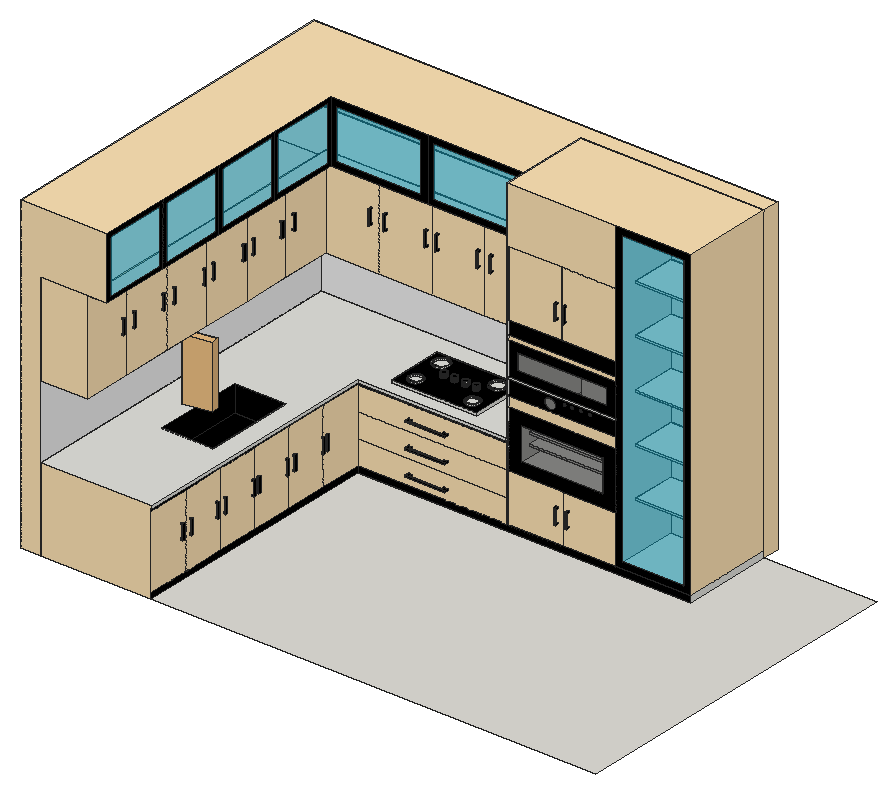
# SketchUp Ruby script. Lengths in inches.
U = 1.inch
M = Sketchup.active_model
def pt(a) = Geom::Point3d.new(a.map { |v| v * U })
def face(e, loops, mat)
  f = e.add_face(loops[0].map { |a| pt(a) })
  loops[1..].each { |l| e.add_face(l.map { |a| pt(a) }).erase! }
  f.material = f.back_material = mat if mat
  f
end
# faces: each face lists its corners as indices into pts; further lists are holes
def faces(e, pts, list, mat = nil) = list.each { |f| face(e, (f[0].is_a?(Array) ? f : [f]).map { |l| l.map { |i| pts[i] } }, mat) }
# xy, xz, yz: faces in a plane at the given z, y or x. An outline is a flat list of corners, or four numbers for a rectangle; further outlines are holes
def ring(l) = l.size == 4 ? [[l[0], l[1]], [l[2], l[1]], [l[2], l[3]], [l[0], l[3]]] : l.each_slice(2).to_a
def flat(e, list, mat, &to3) = list.each { |f| face(e, (f[0].is_a?(Array) ? f : [f]).map { |l| ring(l).map { |u, v| to3.(u, v) } }, mat) }
def xy(e, z, list, mat = nil) = flat(e, list, mat) { |x, y| [x, y, z] }
def xz(e, y, list, mat = nil) = flat(e, list, mat) { |x, z| [x, y, z] }
def yz(e, x, list, mat = nil) = flat(e, list, mat) { |y, z| [x, y, z] }
def lines(e, pts, list) = list.each { |a, b| e.add_line(pt(pts[a]), pt(pts[b])) }
# prism: a flat outline (further loops are holes) pulled along v
def prism(e, loops, v, mat = nil)
  f = face(e, loops, mat); d = Geom::Vector3d.new(v.map { |x| x * U })
  f.pushpull(f.normal.samedirection?(d) ? d.length : -d.length)
end
def box(e, o, s, mat = nil) = prism(e, [[o, [o[0] + s[0], o[1], o[2]], [o[0] + s[0], o[1] + s[1], o[2]], [o[0], o[1] + s[1], o[2]]]], [0, 0, s[2]], mat)
def at(x, y, z, deg = 0) = Geom::Transformation.translation(pt([x, y, z])) * Geom::Transformation.rotation(ORIGIN, Z_AXIS, deg.degrees)
def axes(o, x, y, z) = Geom::Transformation.new([*x, 0, *y, 0, *z, 0, *pt(o).to_a, 1])
def part(name) = M.definitions.add(name)
# library, detail: a bought-in or finely detailed component or shape, given as its bounding box
def library(name, o, s) = part(name).tap { |d| box(d.entities, o, s) }
def detail(e, o, s) = box(e.add_group.entities, o, s)
def put(e, d, t, mat = nil) = e.add_instance(d, t).tap { |i| i.material = mat if mat }
def group(e, t, mat = nil) = e.add_group.tap { |g| g.transformation = t; g.material = mat if mat }.entities
root = M.entities
M.materials.add("[0032_Moccasin]").color = [255, 228, 181]
M.materials.add("[0137_Black]").color = [0, 0, 0]
M.materials.add("[Carrera Marble]").color = [239, 239, 239]
M.materials.add("[Marble Carrara Gold Floor Tile]").color = [225, 223, 217]
M.materials.add("[Translucent Glass Gray]").color = [53, 53, 53]
M.materials["[Translucent Glass Gray]"].alpha = 0.5
M.materials.add("[Translucent Glass Tinted]").color = [7, 187, 224]
M.materials["[Translucent Glass Tinted]"].alpha = 0.48
c1 = part("Group\#2")
xy(c1.entities,0,[[0,0,0.375,0.22]])
xy(c1.entities,0.1875,[[0,0,0.27,0.22]])
xy(c1.entities,1.75,[[0,0,0.27,0.22]])
xy(c1.entities,1.9375,[[0,0,0.375,0.22]])
xz(c1.entities,0,[[0,0,0.375,0,0.375,1.9375,0,1.9375,0,1.75,0.27,1.75,0.27,0.1875,0,0.1875]])
xz(c1.entities,0.22,[[0,0,0,0.1875,0.27,0.1875,0.27,1.75,0,1.75,0,1.9375,0.375,1.9375,0.375,0]])
yz(c1.entities,0.27,[[0,0.1875,0.22,1.75]])
yz(c1.entities,0.375,[[0,0,0.22,1.9375]])
c2 = library("Group\#3",[0,0,0],[12,29.06,81.36])
xy(root,0,[[0,0,0,46.44,58.57,46.44,58.57,44.34,2.55,44.34,2.55,0],[2.55,0,2.55,44.34,58.57,44.34,58.57,32.6875,16.51,32.6875,16.51,0]])
xy(root,0,[[16.51,0,72.74,0,72.74,44.34,58.57,44.34,58.57,32.6875,16.51,32.6875]],"[Marble Carrara Gold Floor Tile]")
xy(root,0.74,[[35.38,32.6875,58.57,44.34]])
xy(root,1.6,[[50.01,32.6875,57.71,40.25]])
xy(root,7.25,[[7.58,12.86,14.08,24.36]],"[0137_Black]")
xy(root,7.76,[[50.01,34.625,57.71,40.25]])
xy(root,7.99,[[50.01,34.625,57.71,40.25]])
xy(root,8.47,[[37.24,32.6875,47.54,36.6875]])
xy(root,9.82,[[37.24,33.8125,47.54,36.6875]])
xy(root,10.05,[[37.24,33.8125,47.54,36.6875]])
xy(root,10.25,[[16.51,0,16.51,32.6875,35.38,32.6875,35.38,32.5625,16.64,32.5625,16.64,0]])
xy(root,10.5625,[[[2.55,0,16.64,0,16.64,32.5625,35.38,32.5625,35.38,44.34,2.55,44.34],[19.61,34.25,30.3,41.32],[7.58,12.86,14.08,24.36]],[19.61,34.25,30.3,41.32]])
xy(root,10.9375,[[[21.41,34.87,21.19,34.9,20.97,34.99,20.79,35.125,20.65,35.31,20.57,35.52,20.54,35.74,20.57,35.97,20.65,36.18,20.79,36.36,20.97,36.5,21.19,36.59,21.41,36.62,21.64,36.59,21.85,36.5,22.03,36.36,22.17,36.18,22.26,35.97,22.29,35.74,22.26,35.52,22.17,35.31,22.03,35.125,21.85,34.99,21.64,34.9],[21.41,35.04,21.59,35.07,21.76,35.14,21.91,35.25,22.02,35.39,22.09,35.5625,22.11,35.74,22.09,35.92,22.02,36.09,21.91,36.24,21.76,36.35,21.59,36.42,21.41,36.44,21.23,36.42,21.0625,36.35,20.92,36.24,20.8,36.09,20.73,35.92,20.71,35.74,20.73,35.5625,20.8,35.39,20.92,35.25,21.0625,35.14,21.23,35.07]],[[28.6,34.87,28.375,34.9,28.16,34.99,27.98,35.125,27.84,35.31,27.75,35.52,27.72,35.74,27.75,35.97,27.84,36.18,27.98,36.36,28.16,36.5,28.375,36.59,28.6,36.62,28.83,36.59,29.04,36.5,29.22,36.36,29.36,36.18,29.44,35.97,29.47,35.74,29.44,35.52,29.36,35.31,29.22,35.125,29.04,34.99,28.83,34.9],[28.6,35.0625,28.78,35.08,28.94,35.15,29.08,35.26,29.19,35.4,29.26,35.57,29.28,35.74,29.26,35.92,29.19,36.08,29.08,36.22,28.94,36.33,28.78,36.4,28.6,36.42,28.42,36.4,28.26,36.33,28.12,36.22,28.01,36.08,27.94,35.92,27.92,35.74,27.94,35.57,28.01,35.4,28.12,35.26,28.26,35.15,28.42,35.08]],[21.41,35.04,21.59,35.07,21.76,35.14,21.91,35.25,22.02,35.39,22.09,35.5625,22.11,35.74,22.09,35.92,22.02,36.09,21.91,36.24,21.76,36.35,21.59,36.42,21.41,36.44,21.23,36.42,21.0625,36.35,20.92,36.24,20.8,36.09,20.73,35.92,20.71,35.74,20.73,35.5625,20.8,35.39,20.92,35.25,21.0625,35.14,21.23,35.07],[28.6,35.0625,28.78,35.08,28.94,35.15,29.08,35.26,29.19,35.4,29.26,35.57,29.28,35.74,29.26,35.92,29.19,36.08,29.08,36.22,28.94,36.33,28.78,36.4,28.6,36.42,28.42,36.4,28.26,36.33,28.12,36.22,28.01,36.08,27.94,35.92,27.92,35.74,27.94,35.57,28.01,35.4,28.12,35.26,28.26,35.15,28.42,35.08],[23.23,37.54,23.14,37.56,23.05,37.59,22.97,37.65,22.91,37.73,22.87,37.82,22.86,37.92,22.87,38.02,22.91,38.11,22.97,38.18,23.05,38.24,23.14,38.28,23.23,38.29,23.33,38.28,23.42,38.24,23.5,38.18,23.56,38.11,23.6,38.02,23.61,37.92,23.6,37.82,23.56,37.73,23.5,37.65,23.42,37.59,23.33,37.56],
  [24.56,37.54,24.46,37.56,24.37,37.59,24.29,37.65,24.23,37.73,24.2,37.82,24.18,37.92,24.2,38.02,24.23,38.11,24.29,38.18,24.37,38.24,24.46,38.28,24.56,38.29,24.65,38.28,24.74,38.24,24.82,38.18,24.88,38.11,24.92,38.02,24.93,37.92,24.92,37.82,24.88,37.73,24.82,37.65,24.74,37.59,24.65,37.56],[25.95,37.54,25.85,37.56,25.76,37.6,25.6875,37.66,25.63,37.74,25.59,37.83,25.58,37.93,25.6,38.03,25.64,38.12,25.7,38.19,25.78,38.25,25.87,38.28,25.97,38.29,26.07,38.28,26.16,38.24,26.23,38.18,26.29,38.1,26.32,38.01,26.33,37.91,26.32,37.8125,26.28,37.72,26.22,37.65,26.14,37.59,26.05,37.55],[27.3125,37.55,27.22,37.57,27.13,37.6,27.06,37.66,27,37.74,26.96,37.82,26.95,37.92,26.96,38.01,27,38.1,27.06,38.18,27.13,38.23,27.22,38.27,27.3125,38.28,27.41,38.27,27.5,38.23,27.57,38.18,27.63,38.1,27.67,38.01,27.68,37.92,27.67,37.82,27.63,37.74,27.57,37.66,27.5,37.6,27.41,37.57],[[28.67,38.77,28.41,38.79,28.17,38.87,27.95,39.01,27.77,39.21,27.66,39.44,27.6,39.7,27.62,39.96,27.7,40.21,27.84,40.42,28.04,40.6,28.27,40.72,28.53,40.77,28.79,40.75,29.03,40.67,29.25,40.53,29.43,40.33,29.54,40.1,29.6,39.85,29.58,39.59,29.5,39.34,29.36,39.12,29.16,38.95,28.93,38.83],[28.66,38.97,28.87,39.01,29.05,39.11,29.21,39.25,29.33,39.42,29.39,39.62,29.4,39.83,29.36,40.04,29.27,40.23,29.125,40.38,28.95,40.5,28.75,40.5625,28.54,40.58,28.33,40.53,28.15,40.4375,27.99,40.3,27.875,40.12,27.81,39.92,27.8,39.71,27.84,39.51,27.93,39.32,28.07,39.16,28.25,39.05,28.45,38.98]],[[21.27,38.78,21.02,38.85,20.79,38.99,20.61,39.17,20.48,39.4,20.42,39.65,20.42,39.91,20.49,40.16,20.625,40.39,20.8125,40.57,21.04,40.7,21.29,40.76,21.55,40.76,21.8,40.69,22.03,40.56,22.21,40.37,22.34,40.14,22.4,39.89,22.4,39.63,22.33,39.38,22.2,39.15,22.01,38.97,21.78,38.84,21.53,38.78],[21.29,38.95,21.51,38.95,21.72,39,21.91,39.11,22.0625,39.26,22.17,39.45,22.23,39.66,22.23,39.87,22.18,40.08,22.07,40.27,21.92,40.42,21.74,40.53,21.53,40.59,21.3125,40.59,21.1,40.54,20.92,40.43,20.76,40.28,20.65,40.1,20.59,39.89,20.59,39.67,20.64,39.46,20.75,39.28,20.9,39.12,21.09,39.01]],
  [21.29,38.95,21.51,38.95,21.72,39,21.91,39.11,22.0625,39.26,22.17,39.45,22.23,39.66,22.23,39.87,22.18,40.08,22.07,40.27,21.92,40.42,21.74,40.53,21.53,40.59,21.3125,40.59,21.1,40.54,20.92,40.43,20.76,40.28,20.65,40.1,20.59,39.89,20.59,39.67,20.64,39.46,20.75,39.28,20.9,39.12,21.09,39.01],[28.66,38.97,28.87,39.01,29.05,39.11,29.21,39.25,29.33,39.42,29.39,39.62,29.4,39.83,29.36,40.04,29.27,40.23,29.125,40.38,28.95,40.5,28.75,40.5625,28.54,40.58,28.33,40.53,28.15,40.4375,27.99,40.3,27.875,40.12,27.81,39.92,27.8,39.71,27.84,39.51,27.93,39.32,28.07,39.16,28.25,39.05,28.45,38.98]])
xy(root,10.9375,[[[19.61,34.25,30.3,41.32],[28.67,38.77,28.41,38.79,28.17,38.87,27.95,39.01,27.77,39.21,27.66,39.44,27.6,39.7,27.62,39.96,27.7,40.21,27.84,40.42,28.04,40.6,28.27,40.72,28.53,40.77,28.79,40.75,29.03,40.67,29.25,40.53,29.43,40.33,29.54,40.1,29.6,39.85,29.58,39.59,29.5,39.34,29.36,39.12,29.16,38.95,28.93,38.83],[21.27,38.78,21.02,38.85,20.79,38.99,20.61,39.17,20.48,39.4,20.42,39.65,20.42,39.91,20.49,40.16,20.625,40.39,20.8125,40.57,21.04,40.7,21.29,40.76,21.55,40.76,21.8,40.69,22.03,40.56,22.21,40.37,22.34,40.14,22.4,39.89,22.4,39.63,22.33,39.38,22.2,39.15,22.01,38.97,21.78,38.84,21.53,38.78],[21.41,34.87,21.19,34.9,20.97,34.99,20.79,35.125,20.65,35.31,20.57,35.52,20.54,35.74,20.57,35.97,20.65,36.18,20.79,36.36,20.97,36.5,21.19,36.59,21.41,36.62,21.64,36.59,21.85,36.5,22.03,36.36,22.17,36.18,22.26,35.97,22.29,35.74,22.26,35.52,22.17,35.31,22.03,35.125,21.85,34.99,21.64,34.9],[28.6,34.87,28.375,34.9,28.16,34.99,27.98,35.125,27.84,35.31,27.75,35.52,27.72,35.74,27.75,35.97,27.84,36.18,27.98,36.36,28.16,36.5,28.375,36.59,28.6,36.62,28.83,36.59,29.04,36.5,29.22,36.36,29.36,36.18,29.44,35.97,29.47,35.74,29.44,35.52,29.36,35.31,29.22,35.125,29.04,34.99,28.83,34.9],[25.95,37.54,25.85,37.56,25.76,37.6,25.6875,37.66,25.63,37.74,25.59,37.83,25.58,37.93,25.6,38.03,25.64,38.12,25.7,38.19,25.78,38.25,25.87,38.28,25.97,38.29,26.07,38.28,26.16,38.24,26.23,38.18,26.29,38.1,26.32,38.01,26.33,37.91,26.32,37.8125,26.28,37.72,26.22,37.65,26.14,37.59,26.05,37.55],[23.23,37.54,23.14,37.56,23.05,37.59,22.97,37.65,22.91,37.73,22.87,37.82,22.86,37.92,22.87,38.02,22.91,38.11,22.97,38.18,23.05,38.24,23.14,38.28,23.23,38.29,23.33,38.28,23.42,38.24,23.5,38.18,23.56,38.11,23.6,38.02,23.61,37.92,23.6,37.82,23.56,37.73,23.5,37.65,23.42,37.59,23.33,37.56],[24.56,37.54,24.46,37.56,24.37,37.59,24.29,37.65,24.23,37.73,24.2,37.82,24.18,37.92,24.2,38.02,24.23,38.11,24.29,38.18,24.37,38.24,24.46,38.28,24.56,38.29,24.65,38.28,24.74,38.24,24.82,38.18,24.88,38.11,24.92,38.02,24.93,37.92,24.92,37.82,24.88,37.73,24.82,37.65,24.74,37.59,24.65,37.56],[27.3125,37.55,27.22,37.57,27.13,37.6,27.06,37.66,27,37.74,26.96,37.82,26.95,37.92,26.96,38.01,27,38.1,27.06,38.18,27.13,38.23,27.22,38.27,27.3125,38.28,27.41,38.27,27.5,38.23,27.57,38.18,27.63,38.1,27.67,38.01,27.68,37.92,27.67,37.82,27.63,37.74,27.57,37.66,27.5,37.6,27.41,37.57]]],"[0137_Black]")
xy(root,11.0625,[[[21.41,34.87,21.64,34.9,21.85,34.99,22.03,35.125,22.17,35.31,22.26,35.52,22.29,35.74,22.26,35.97,22.17,36.18,22.03,36.36,21.85,36.5,21.64,36.59,21.41,36.62,21.19,36.59,20.97,36.5,20.79,36.36,20.65,36.18,20.57,35.97,20.54,35.74,20.57,35.52,20.65,35.31,20.79,35.125,20.97,34.99,21.19,34.9],[21.41,35.04,21.23,35.07,21.0625,35.14,20.92,35.25,20.8,35.39,20.73,35.5625,20.71,35.74,20.73,35.92,20.8,36.09,20.92,36.24,21.0625,36.35,21.23,36.42,21.41,36.44,21.59,36.42,21.76,36.35,21.91,36.24,22.02,36.09,22.09,35.92,22.11,35.74,22.09,35.5625,22.02,35.39,21.91,35.25,21.76,35.14,21.59,35.07]],[[28.6,34.87,28.83,34.9,29.04,34.99,29.22,35.125,29.36,35.31,29.44,35.52,29.47,35.74,29.44,35.97,29.36,36.18,29.22,36.36,29.04,36.5,28.83,36.59,28.6,36.62,28.375,36.59,28.16,36.5,27.98,36.36,27.84,36.18,27.75,35.97,27.72,35.74,27.75,35.52,27.84,35.31,27.98,35.125,28.16,34.99,28.375,34.9],[28.6,35.0625,28.42,35.08,28.26,35.15,28.12,35.26,28.01,35.4,27.94,35.57,27.92,35.74,27.94,35.92,28.01,36.08,28.12,36.22,28.26,36.33,28.42,36.4,28.6,36.42,28.78,36.4,28.94,36.33,29.08,36.22,29.19,36.08,29.26,35.92,29.28,35.74,29.26,35.57,29.19,35.4,29.08,35.26,28.94,35.15,28.78,35.08]],[[28.67,38.77,28.93,38.83,29.16,38.95,29.36,39.12,29.5,39.34,29.58,39.59,29.6,39.85,29.54,40.1,29.43,40.33,29.25,40.53,29.03,40.67,28.79,40.75,28.53,40.77,28.27,40.72,28.04,40.6,27.84,40.42,27.7,40.21,27.62,39.96,27.6,39.7,27.66,39.44,27.77,39.21,27.95,39.01,28.17,38.87,28.41,38.79],[28.66,38.97,28.45,38.98,28.25,39.05,28.07,39.16,27.93,39.32,27.84,39.51,27.8,39.71,27.81,39.92,27.875,40.12,27.99,40.3,28.15,40.4375,28.33,40.53,28.54,40.58,28.75,40.5625,28.95,40.5,29.125,40.38,29.27,40.23,29.36,40.04,29.4,39.83,29.39,39.62,29.33,39.42,29.21,39.25,29.05,39.11,28.87,39.01]],[[21.27,38.78,21.53,38.78,21.78,38.84,22.01,38.97,22.2,39.15,22.33,39.38,22.4,39.63,22.4,39.89,22.34,40.14,22.21,40.37,22.03,40.56,21.8,40.69,21.55,40.76,21.29,40.76,21.04,40.7,20.8125,40.57,20.625,40.39,20.49,40.16,20.42,39.91,20.42,39.65,20.48,39.4,20.61,39.17,20.79,38.99,21.02,38.85],[21.29,38.95,21.09,39.01,20.9,39.12,20.75,39.28,20.64,39.46,20.59,39.67,20.59,39.89,20.65,40.1,20.76,40.28,20.92,40.43,21.1,40.54,21.3125,40.59,21.53,40.59,21.74,40.53,21.92,40.42,22.07,40.27,22.18,40.08,22.23,39.87,22.23,39.66,22.17,39.45,22.0625,39.26,21.91,39.11,21.72,39,21.51,38.95]]],"[0137_Black]")
xy(root,11.16,[[37.24,33.8125,47.54,36.6875]])
xy(root,11.36,[[37.24,33.8125,47.54,36.6875]])
xy(root,11.4375,[[23.23,37.54,23.33,37.56,23.42,37.59,23.5,37.65,23.56,37.73,23.6,37.82,23.61,37.92,23.6,38.02,23.56,38.11,23.5,38.18,23.42,38.24,23.33,38.28,23.23,38.29,23.14,38.28,23.05,38.24,22.97,38.18,22.91,38.11,22.87,38.02,22.86,37.92,22.87,37.82,22.91,37.73,22.97,37.65,23.05,37.59,23.14,37.56],[24.56,37.54,24.65,37.56,24.74,37.59,24.82,37.65,24.88,37.73,24.92,37.82,24.93,37.92,24.92,38.02,24.88,38.11,24.82,38.18,24.74,38.24,24.65,38.28,24.56,38.29,24.46,38.28,24.37,38.24,24.29,38.18,24.23,38.11,24.2,38.02,24.18,37.92,24.2,37.82,24.23,37.73,24.29,37.65,24.37,37.59,24.46,37.56],[25.95,37.54,26.05,37.55,26.14,37.59,26.22,37.65,26.28,37.72,26.32,37.8125,26.33,37.91,26.32,38.01,26.29,38.1,26.23,38.18,26.16,38.24,26.07,38.28,25.97,38.29,25.87,38.28,25.78,38.25,25.7,38.19,25.64,38.12,25.6,38.03,25.58,37.93,25.59,37.83,25.63,37.74,25.6875,37.66,25.76,37.6,25.85,37.56],[27.3125,37.55,27.41,37.57,27.5,37.6,27.57,37.66,27.63,37.74,27.67,37.82,27.68,37.92,27.67,38.01,27.63,38.1,27.57,38.18,27.5,38.23,27.41,38.27,27.3125,38.28,27.22,38.27,27.13,38.23,27.06,38.18,27,38.1,26.96,38.01,26.95,37.92,26.96,37.82,27,37.74,27.06,37.66,27.13,37.6,27.22,37.57]],"[0137_Black]")
xy(root,12.51,[[37.24,32.6875,47.54,36.6875]])
xy(root,13.91,[[50.01,34.625,57.71,40.25]])
xy(root,14.15,[[50.01,34.625,57.71,40.25]])
xy(root,19.85,[[2.55,0,2.55,44.34,35.38,44.34,35.38,37.65,8.49,37.65,8.49,0]])
xy(root,20.06,[[50.01,34.625,57.71,40.25]])
xy(root,20.3,[[50.01,34.625,57.71,40.25]])
xy(root,24.01,[[35.56,32.6875,35.64,32.75],[42.25,32.6875,42.28,32.75]])
xy(root,26.21,[[50.01,34.625,57.71,40.25]])
xy(root,26.45,[[50.01,34.625,57.71,40.25]])
xy(root,31.56,[[2.55,0,8.49,36.47],[8.49,0,8.49,37.65,35.38,37.65,35.38,35.34,10.99,35.34,10.99,0],[2.55,36.47,8.49,36.47,8.49,37.65,35.38,37.65,35.38,44.34,2.55,44.34]])
xy(root,32.29,[[35.56,32.6875,35.64,32.75],[42.25,32.6875,42.28,32.75]])
xy(root,32.36,[[50.01,34.625,57.71,40.25]])
xy(root,32.6,[[50.01,34.625,57.71,40.25]])
xy(root,38.51,[[50.01,32.6875,57.71,40.25]])
xy(root,39.375,[[0,0,10.99,0,10.99,35.34,35.38,35.34,35.38,44.34,58.57,44.34,58.57,46.44,0,46.44],[35.38,32.6875,58.57,44.34]],"[0032_Moccasin]")
xz(root,0,[[0,0,2.55,0,2.55,31.56,10.99,31.56,10.99,39.375,0,39.375],[2.55,0,16.51,0,16.51,10.25,16.64,10.25,16.64,10.5625,2.55,10.5625],[2.55,19.85,8.49,31.56]],"[0032_Moccasin]")
xz(root,12.86,[[7.58,7.25,14.08,10.5625]],"[0137_Black]")
xz(root,24.36,[[7.58,7.25,14.08,10.5625]],"[0137_Black]")
xz(root,32.5625,[[16.64,10.25,35.38,10.5625]])
xz(root,32.6875,[[35.38,0.74,35.64,24.01],[35.64,17.33,49.14,17.52],[35.38,24.01,35.56,32.29]])
xz(root,32.6875,[[16.51,0.74,35.38,3.8],[35.64,0.74,42.39,6.86],[42.39,0.74,49.14,6.86],[16.51,3.8,35.38,6.86],[16.51,6.86,35.38,9.92],
  [35.64,14.11,49.14,15.4375],[35.64,21.77,49.14,22.3],[35.64,24.01,42.25,32.29],[42.28,24.01,49.14,32.29],[35.38,32.29,49.14,39.375]],"[0032_Moccasin]")
xz(root,32.6875,[[16.51,0,58.57,0.74],[[49.14,0.74,58.57,39.375],[50.01,1.6,57.71,38.51]],[[35.64,6.86,49.14,14.11],[37.24,8.47,47.54,12.51]],[16.51,9.92,35.38,10.25],[[35.64,15.4375,49.14,17.33],[40.85,15.62,40.68,15.64,40.51,15.71,40.37,15.82,40.26,15.96,40.1875,16.13,40.17,16.31,40.1875,16.49,40.26,16.65,40.37,16.79,40.51,16.9,40.68,16.97,40.85,17,41.03,16.97,41.2,16.9,41.34,16.79,41.45,16.65,41.52,16.49,41.54,16.31,41.52,16.13,41.45,15.96,41.34,15.82,41.2,15.71,41.03,15.64],[43.66,16.62,43.61,16.625,43.5625,16.64,43.52,16.67,43.49,16.71,43.47,16.76,43.47,16.85,43.49,16.9,43.52,16.9375,43.5625,16.97,43.61,16.99,43.7,16.99,43.75,16.97,43.79,16.9375,43.82,16.9,43.84,16.85,43.84,16.76,43.82,16.71,43.79,16.67,43.75,16.64,43.7,16.625],[45.9,16.62,45.85,16.625,45.81,16.64,45.77,16.67,45.74,16.71,45.72,16.76,45.72,16.85,45.74,16.9,45.77,16.9375,45.81,16.97,45.85,16.99,45.95,16.99,46,16.97,46.04,16.9375,46.07,16.9,46.08,16.85,46.09,16.81,46.07,16.71,46.04,16.67,46,16.64,45.95,16.625],[44.74,16.62,44.69,16.625,44.65,16.64,44.61,16.67,44.58,16.71,44.5625,16.76,44.56,16.81,44.5625,16.85,44.58,16.9,44.61,16.9375,44.65,16.97,44.69,16.99,44.79,16.99,44.84,16.97,44.875,16.9375,44.91,16.9,44.92,16.85,44.93,16.81,44.91,16.71,44.875,16.67,44.84,16.64,44.79,16.625],[42.7,16.62,42.65,16.625,42.61,16.64,42.57,16.67,42.54,16.71,42.52,16.76,42.51,16.81,42.52,16.85,42.54,16.9,42.57,16.9375,42.61,16.97,42.65,16.99,42.75,16.99,42.8,16.97,42.83,16.9375,42.86,16.9,42.88,16.85,42.89,16.81,42.88,16.76,42.86,16.71,42.83,16.67,42.8,16.64,42.75,16.625]],
  [[35.64,17.52,49.14,21.77],[36.73,18.62,48.05,20.68]],[35.64,22.3,49.14,24.01]],"[0137_Black]")
xz(root,32.6875,[[37.24,8.47,47.54,12.51],[40.85,15.62,41.03,15.64,41.2,15.71,41.34,15.82,41.45,15.96,41.52,16.13,41.54,16.31,41.52,16.49,41.45,16.65,41.34,16.79,41.2,16.9,41.03,16.97,40.85,17,40.68,16.97,40.51,16.9,40.37,16.79,40.26,16.65,40.1875,16.49,40.17,16.31,40.1875,16.13,40.26,15.96,40.37,15.82,40.51,15.71,40.68,15.64],[42.7,16.62,42.75,16.625,42.8,16.64,42.83,16.67,42.86,16.71,42.88,16.76,42.89,16.81,42.88,16.85,42.86,16.9,42.83,16.9375,42.8,16.97,42.75,16.99,42.65,16.99,42.61,16.97,42.57,16.9375,42.54,16.9,42.52,16.85,42.51,16.81,42.52,16.76,42.54,16.71,42.57,16.67,42.61,16.64,42.65,16.625],[43.66,16.62,43.7,16.625,43.75,16.64,43.79,16.67,43.82,16.71,43.84,16.76,43.84,16.85,43.82,16.9,43.79,16.9375,43.75,16.97,43.7,16.99,43.61,16.99,43.5625,16.97,43.52,16.9375,43.49,16.9,43.47,16.85,43.47,16.76,43.49,16.71,43.52,16.67,43.5625,16.64,43.61,16.625],[44.74,16.62,44.79,16.625,44.84,16.64,44.875,16.67,44.91,16.71,44.93,16.81,44.92,16.85,44.91,16.9,44.875,16.9375,44.84,16.97,44.79,16.99,44.69,16.99,44.65,16.97,44.61,16.9375,44.58,16.9,44.5625,16.85,44.56,16.81,44.5625,16.76,44.58,16.71,44.61,16.67,44.65,16.64,44.69,16.625],
  [45.9,16.62,45.95,16.625,46,16.64,46.04,16.67,46.07,16.71,46.09,16.81,46.08,16.85,46.07,16.9,46.04,16.9375,46,16.97,45.95,16.99,45.85,16.99,45.81,16.97,45.77,16.9375,45.74,16.9,45.72,16.85,45.72,16.76,45.74,16.71,45.77,16.67,45.81,16.64,45.85,16.625],[36.73,18.62,48.05,20.68]],"[Translucent Glass Gray]")
xz(root,32.6875,[[50.01,1.6,57.71,38.51]],"[Translucent Glass Tinted]")
xz(root,32.75,[[35.56,24.01,35.64,32.29],[42.25,24.01,42.28,32.29]])
xz(root,33.8125,[[37.24,9.82,47.54,10.05],[37.24,11.16,47.54,11.36]])
xz(root,34.25,[[19.61,10.5625,30.3,10.9375]])
xz(root,34.625,[[50.01,7.76,57.71,7.99],[50.01,13.91,57.71,14.15],[50.01,20.06,57.71,20.3],[50.01,26.21,57.71,26.45],[50.01,32.36,57.71,32.6]])
xz(root,35.34,[[[10.99,31.56,23.1875,39.375],[11.75,32.32,22.42,38.61]],[[23.1875,31.56,35.38,39.375],[23.95,32.32,34.62,38.61]]],"[0137_Black]")
xz(root,35.34,[[11.75,32.32,22.42,38.61],[23.95,32.32,34.62,38.61]],"[Translucent Glass Tinted]")
xz(root,36.6875,[[37.24,8.47,47.54,9.82],[37.24,10.05,47.54,11.16],[37.24,11.16,47.54,11.36],[37.24,11.36,47.54,12.51]])
xz(root,37.65,[[8.49,19.85,15.21,31.56],[15.21,19.85,21.9375,31.56],[21.9375,19.85,28.66,31.56],[28.66,19.85,35.38,31.56]],"[0032_Moccasin]")
xz(root,38.78,[[21.27,10.9375,21.53,11.0625]])
xz(root,38.95,[[21.29,10.9375,21.51,11.0625]])
xz(root,40.25,[[50.01,1.6,57.71,7.76],[50.01,7.76,57.71,7.99],[50.01,7.99,57.71,13.91],[50.01,13.91,57.71,14.15],[50.01,14.15,57.71,20.06],
  [50.01,20.06,57.71,20.3],[50.01,20.3,57.71,26.21],[50.01,26.21,57.71,26.45],[50.01,26.45,57.71,32.36],[50.01,32.36,57.71,32.6],
  [50.01,32.6,57.71,38.51]])
xz(root,40.59,[[21.3125,10.9375,21.53,11.0625]])
xz(root,40.76,[[21.29,10.9375,21.55,11.0625]])
xz(root,41.32,[[19.61,10.5625,30.3,10.9375]])
xz(root,44.34,[[2.55,0,58.57,0,58.57,0.74,35.38,0.74,35.38,10.5625,2.55,10.5625],[35.38,0.74,58.57,39.375],[2.55,19.85,35.38,31.56]])
xz(root,44.34,[[2.55,10.5625,35.38,19.85]],"[Carrera Marble]")
xz(root,46.44,[[0,0,58.57,39.375]])
yz(root,0,[[0,0,46.44,39.375]])
yz(root,2.55,[[0,0,44.34,10.5625],[0,19.85,40.34,31.56],[40.34,19.85,44.34,31.56]])
yz(root,2.55,[[0,10.5625,44.34,19.85]],"[Carrera Marble]")
yz(root,7.58,[[12.86,7.25,24.36,10.5625]],"[0137_Black]")
yz(root,8.49,[[0,19.85,6.28,31.56],[6.28,19.85,12.55,31.56],[12.55,19.85,18.83,31.56],[18.83,19.85,25.1,31.56],[25.1,19.85,31.38,31.56],
  [31.38,19.85,37.65,31.56]],"[0032_Moccasin]")
yz(root,10.99,[[[0,31.56,8.84,39.375],[0.53,32.09,8.31,38.85]],[[8.84,31.56,17.67,39.375],[9.36,32.09,17.14,38.85]],[[17.67,31.56,26.51,39.375],[18.2,32.09,25.98,38.85]],[[26.51,31.56,35.34,39.375],[27.03,32.09,34.82,38.85]]],"[0137_Black]")
yz(root,10.99,[[0.53,32.09,8.31,38.85],[9.36,32.09,17.14,38.85],[18.2,32.09,25.98,38.85],[27.03,32.09,34.82,38.85]],"[Translucent Glass Tinted]")
yz(root,14.08,[[12.86,7.25,24.36,10.5625]])
yz(root,16.51,[[4.61,4.73,4.83,4.92],[4.61,6.48,4.83,6.67]])
yz(root,16.51,[[[0,0.74,5.45,9.92],[4.61,6.48,4.83,6.67],[4.61,4.73,4.83,4.92]],[5.45,0.74,10.9,9.92],[10.9,0.74,16.34,9.92],[16.34,0.74,21.79,9.92],[21.79,0.74,27.24,9.92],
  [27.24,0.74,32.6875,9.92]],"[0032_Moccasin]")
yz(root,16.51,[[0,0,32.6875,0.74],[0,9.92,32.6875,10.25]],"[0137_Black]")
yz(root,16.64,[[0,10.25,32.5625,10.5625]])
yz(root,19.61,[[34.25,10.5625,41.32,10.9375]])
yz(root,20.42,[[39.65,10.9375,39.91,11.0625]])
yz(root,20.59,[[39.67,10.9375,39.89,11.0625]])
yz(root,22.23,[[39.66,10.9375,39.87,11.0625]])
yz(root,22.4,[[39.63,10.9375,39.89,11.0625]])
yz(root,30.3,[[34.25,10.5625,41.32,10.9375]])
yz(root,35.38,[[32.6875,0.74,44.34,10.5625],[32.5625,10.25,32.6875,10.5625],[32.6875,10.5625,32.6875,39.375,35.34,39.375,35.34,31.56,37.65,31.56,37.65,19.85,44.34,19.85,44.34,10.5625],[37.65,19.85,44.34,31.56],[35.34,31.56,44.34,39.375]])
yz(root,35.56,[[32.6875,24.01,32.75,32.29]])
yz(root,35.64,[[32.6875,24.01,32.75,32.29]])
yz(root,37.24,[[32.6875,8.47,36.6875,8.47,36.6875,9.82,33.8125,9.82,33.8125,10.05,36.6875,10.05,36.6875,11.16,33.8125,11.16,33.8125,11.36,36.6875,11.36,36.6875,12.51,32.6875,12.51],[33.8125,11.16,36.6875,11.36]])
yz(root,42.25,[[32.6875,24.01,32.75,32.29]])
yz(root,42.28,[[32.6875,24.01,32.75,32.29]])
yz(root,47.54,[[32.6875,8.47,32.6875,12.51,36.6875,12.51,36.6875,11.36,33.8125,11.36,33.8125,11.16,36.6875,11.16,36.6875,10.05,33.8125,10.05,33.8125,9.82,36.6875,9.82,36.6875,8.47],[33.8125,11.16,36.6875,11.36]])
yz(root,50.01,[[32.6875,1.6,40.25,1.6,40.25,7.76,34.625,7.76,34.625,7.99,40.25,7.99,40.25,13.91,34.625,13.91,34.625,14.15,40.25,14.15,40.25,20.06,34.625,20.06,34.625,20.3,40.25,20.3,40.25,26.21,34.625,26.21,34.625,26.45,40.25,26.45,40.25,32.36,34.625,32.36,34.625,32.6,40.25,32.6,40.25,38.51,32.6875,38.51],[34.625,7.76,40.25,7.99],[34.625,13.91,40.25,14.15],[34.625,20.06,40.25,20.3],[34.625,26.21,40.25,26.45],
  [34.625,32.36,40.25,32.6]])
yz(root,57.71,[[32.6875,1.6,32.6875,38.51,40.25,38.51,40.25,32.6,34.625,32.6,34.625,32.36,40.25,32.36,40.25,26.45,34.625,26.45,34.625,26.21,40.25,26.21,40.25,20.3,34.625,20.3,34.625,20.06,40.25,20.06,40.25,14.15,34.625,14.15,34.625,13.91,40.25,13.91,40.25,7.99,34.625,7.99,34.625,7.76,40.25,7.76,40.25,1.6],[34.625,7.76,40.25,7.99],[34.625,13.91,40.25,14.15],[34.625,20.06,40.25,20.3],[34.625,26.21,40.25,26.45],
  [34.625,32.36,40.25,32.6]])
yz(root,58.57,[[32.6875,0,44.34,0.74]])
yz(root,58.57,[[44.34,0,46.44,39.375],[32.6875,0.74,44.34,39.375]],"[0032_Moccasin]")
p = [[20.97,34.99,10.9375],[21.19,34.9,10.9375],[21.19,34.9,11.0625],[20.97,34.99,11.0625],[21.41,34.87,10.9375],[21.41,34.87,11.0625],
  [21.64,34.9,10.9375],[21.64,34.9,11.0625],[21.85,34.99,10.9375],[21.85,34.99,11.0625],[28.16,34.99,10.9375],[28.375,34.9,10.9375],
  [28.375,34.9,11.0625],[28.16,34.99,11.0625],[28.6,34.87,10.9375],[28.6,34.87,11.0625],[28.83,34.9,10.9375],[28.83,34.9,11.0625],
  [29.04,34.99,10.9375],[29.04,34.99,11.0625],[20.79,35.125,10.9375],[20.79,35.125,11.0625],[21.41,35.04,10.9375],[21.23,35.07,10.9375],
  [21.23,35.07,11.0625],[21.41,35.04,11.0625],[21.59,35.07,10.9375],[21.59,35.07,11.0625],[22.03,35.125,10.9375],[22.03,35.125,11.0625],
  [27.98,35.125,10.9375],[27.98,35.125,11.0625],[29.22,35.125,10.9375],[29.22,35.125,11.0625],[20.65,35.31,10.9375],[20.65,35.31,11.0625],
  [21.0625,35.14,10.9375],[20.92,35.25,10.9375],[20.92,35.25,11.0625],[21.0625,35.14,11.0625],[21.76,35.14,10.9375],[21.76,35.14,11.0625],
  [21.91,35.25,10.9375],[21.91,35.25,11.0625],[22.17,35.31,10.9375],[22.17,35.31,11.0625],[27.84,35.31,10.9375],[27.84,35.31,11.0625],
  [28.42,35.08,10.9375],[28.26,35.15,10.9375],[28.26,35.15,11.0625],[28.42,35.08,11.0625],[28.6,35.0625,10.9375],[28.6,35.0625,11.0625],
  [28.78,35.08,10.9375],[28.78,35.08,11.0625],[28.94,35.15,10.9375],[28.94,35.15,11.0625],[29.36,35.31,10.9375],[29.36,35.31,11.0625],
  [20.8,35.39,10.9375],[20.8,35.39,11.0625],[22.02,35.39,10.9375],[22.02,35.39,11.0625],[28.12,35.26,10.9375],[28.12,35.26,11.0625],
  [29.08,35.26,10.9375],[29.08,35.26,11.0625],[20.57,35.52,10.9375],[20.57,35.52,11.0625],[22.26,35.52,10.9375],[22.26,35.52,11.0625],
  [27.75,35.52,10.9375],[27.75,35.52,11.0625],[28.01,35.4,10.9375],[28.01,35.4,11.0625],[29.19,35.4,10.9375],[29.19,35.4,11.0625],
  [29.44,35.52,10.9375],[29.44,35.52,11.0625],[20.73,35.5625,10.9375],[20.73,35.5625,11.0625],[22.09,35.5625,10.9375],[22.09,35.5625,11.0625],
  [27.94,35.57,10.9375],[27.94,35.57,11.0625],[29.26,35.57,10.9375],[29.26,35.57,11.0625],[20.54,35.74,10.9375],[20.54,35.74,11.0625],
  [22.29,35.74,10.9375],[22.29,35.74,11.0625],[27.72,35.74,10.9375],[27.72,35.74,11.0625],[29.47,35.74,10.9375],[29.47,35.74,11.0625],
  [20.71,35.74,10.9375],[20.71,35.74,11.0625],[22.11,35.74,10.9375],[22.11,35.74,11.0625],[27.92,35.74,10.9375],[27.92,35.74,11.0625],
  [29.28,35.74,10.9375],[29.28,35.74,11.0625],[20.57,35.97,10.9375],[20.57,35.97,11.0625],[20.73,35.92,10.9375],[20.73,35.92,11.0625],
  [22.09,35.92,10.9375],[22.09,35.92,11.0625],[22.26,35.97,10.9375],[22.26,35.97,11.0625],[27.75,35.97,10.9375],[27.75,35.97,11.0625],
  [27.94,35.92,10.9375],[27.94,35.92,11.0625],[29.26,35.92,10.9375],[29.26,35.92,11.0625],[29.44,35.97,10.9375],[29.44,35.97,11.0625],
  [20.8,36.09,10.9375],[20.8,36.09,11.0625],[22.02,36.09,10.9375],[22.02,36.09,11.0625],[28.01,36.08,10.9375],[28.01,36.08,11.0625],
  [29.19,36.08,10.9375],[29.19,36.08,11.0625],[20.65,36.18,10.9375],[20.65,36.18,11.0625],[22.17,36.18,10.9375],[22.17,36.18,11.0625],
  [27.84,36.18,10.9375],[27.84,36.18,11.0625],[29.36,36.18,10.9375],[29.36,36.18,11.0625],[20.92,36.24,10.9375],[20.92,36.24,11.0625],
  [21.91,36.24,10.9375],[21.91,36.24,11.0625],[28.12,36.22,10.9375],[28.12,36.22,11.0625],[29.08,36.22,10.9375],[29.08,36.22,11.0625],
  [20.79,36.36,10.9375],[20.79,36.36,11.0625],[21.0625,36.35,10.9375],[21.0625,36.35,11.0625],[21.76,36.35,10.9375],[21.76,36.35,11.0625],
  [22.03,36.36,10.9375],[22.03,36.36,11.0625],[27.98,36.36,10.9375],[27.98,36.36,11.0625],[28.26,36.33,10.9375],[28.26,36.33,11.0625],
  [28.94,36.33,10.9375],[28.94,36.33,11.0625],[29.22,36.36,10.9375],[29.22,36.36,11.0625],[28.42,36.4,10.9375],[28.42,36.4,11.0625],
  [28.78,36.4,10.9375],[28.78,36.4,11.0625],[20.97,36.5,10.9375],[20.97,36.5,11.0625],[21.23,36.42,10.9375],[21.23,36.42,11.0625],
  [21.41,36.44,10.9375],[21.41,36.44,11.0625],[21.59,36.42,10.9375],[21.59,36.42,11.0625],[21.85,36.5,10.9375],[21.85,36.5,11.0625],
  [28.16,36.5,10.9375],[28.16,36.5,11.0625],[28.6,36.42,10.9375],[28.6,36.42,11.0625],[29.04,36.5,10.9375],[29.04,36.5,11.0625],
  [21.19,36.59,10.9375],[21.19,36.59,11.0625],[21.64,36.59,10.9375],[21.64,36.59,11.0625],[28.375,36.59,10.9375],[28.375,36.59,11.0625],
  [28.83,36.59,10.9375],[28.83,36.59,11.0625],[21.41,36.62,10.9375],[21.41,36.62,11.0625],[28.6,36.62,10.9375],[28.6,36.62,11.0625],
  [23.14,37.56,10.9375],[23.23,37.54,10.9375],[23.23,37.54,11.4375],[23.14,37.56,11.4375],[23.33,37.56,10.9375],[23.33,37.56,11.4375],
  [24.46,37.56,10.9375],[24.56,37.54,10.9375],[24.56,37.54,11.4375],[24.46,37.56,11.4375],[24.65,37.56,10.9375],[24.65,37.56,11.4375],
  [25.85,37.56,10.9375],[25.95,37.54,10.9375],[25.95,37.54,11.4375],[25.85,37.56,11.4375],[26.05,37.55,10.9375],[26.05,37.55,11.4375],
  [23.05,37.59,10.9375],[23.05,37.59,11.4375],[22.97,37.65,10.9375],[22.97,37.65,11.4375],[23.42,37.59,10.9375],[23.42,37.59,11.4375],
  [23.5,37.65,10.9375],[23.5,37.65,11.4375],[24.29,37.65,10.9375],[24.37,37.59,10.9375],[24.37,37.59,11.4375],[24.29,37.65,11.4375],
  [24.74,37.59,10.9375],[24.74,37.59,11.4375],[24.82,37.65,10.9375],[24.82,37.65,11.4375],[25.6875,37.66,10.9375],[25.76,37.6,10.9375],
  [25.76,37.6,11.4375],[25.6875,37.66,11.4375],[26.14,37.59,10.9375],[26.14,37.59,11.4375],[26.22,37.65,10.9375],[26.22,37.65,11.4375],
  [26.28,37.72,10.9375],[26.28,37.72,11.4375],[27.13,37.6,10.9375],[27.22,37.57,10.9375],[27.22,37.57,11.4375],[27.13,37.6,11.4375],
  [27.06,37.66,10.9375],[27.06,37.66,11.4375],[27.3125,37.55,10.9375],[27.3125,37.55,11.4375],[27.41,37.57,10.9375],[27.41,37.57,11.4375],
  [27.5,37.6,10.9375],[27.5,37.6,11.4375],[27.57,37.66,10.9375],[27.57,37.66,11.4375],[22.91,37.73,10.9375],[22.91,37.73,11.4375],
  [22.87,37.82,10.9375],[22.87,37.82,11.4375],[23.56,37.73,10.9375],[23.56,37.73,11.4375],[23.6,37.82,10.9375],[23.6,37.82,11.4375],
  [24.2,37.82,10.9375],[24.23,37.73,10.9375],[24.23,37.73,11.4375],[24.2,37.82,11.4375],[24.88,37.73,10.9375],[24.88,37.73,11.4375],
  [24.92,37.82,10.9375],[24.92,37.82,11.4375],[25.59,37.83,10.9375],[25.63,37.74,10.9375],[25.63,37.74,11.4375],[25.59,37.83,11.4375],
  [26.32,37.8125,10.9375],[26.32,37.8125,11.4375],[26.96,37.82,10.9375],[27,37.74,10.9375],[27,37.74,11.4375],[26.96,37.82,11.4375],
  [27.63,37.74,10.9375],[27.67,37.82,10.9375],[27.67,37.82,11.4375],[27.63,37.74,11.4375],[22.86,37.92,10.9375],[22.86,37.92,11.4375],
  [23.61,37.92,10.9375],[23.61,37.92,11.4375],[24.18,37.92,10.9375],[24.18,37.92,11.4375],[24.93,37.92,10.9375],[24.93,37.92,11.4375],
  [25.58,37.93,10.9375],[25.58,37.93,11.4375],[26.33,37.91,10.9375],[26.33,37.91,11.4375],[26.95,37.92,10.9375],[26.95,37.92,11.4375],
  [27.68,37.92,10.9375],[27.68,37.92,11.4375],[22.87,38.02,10.9375],[22.87,38.02,11.4375],[23.6,38.02,10.9375],[23.6,38.02,11.4375],
  [24.2,38.02,10.9375],[24.2,38.02,11.4375],[24.92,38.02,10.9375],[24.92,38.02,11.4375],[25.6,38.03,10.9375],[25.6,38.03,11.4375],
  [26.32,38.01,10.9375],[26.32,38.01,11.4375],[26.96,38.01,10.9375],[26.96,38.01,11.4375],[27.67,38.01,10.9375],[27.67,38.01,11.4375],
  [22.91,38.11,10.9375],[22.91,38.11,11.4375],[23.56,38.11,10.9375],[23.56,38.11,11.4375],[24.23,38.11,10.9375],[24.23,38.11,11.4375],
  [24.88,38.11,10.9375],[24.88,38.11,11.4375],[25.64,38.12,10.9375],[25.64,38.12,11.4375],[26.29,38.1,10.9375],[26.29,38.1,11.4375],
  [27,38.1,10.9375],[27,38.1,11.4375],[27.63,38.1,10.9375],[27.63,38.1,11.4375],[22.97,38.18,10.9375],[22.97,38.18,11.4375],
  [23.5,38.18,10.9375],[23.5,38.18,11.4375],[24.29,38.18,10.9375],[24.29,38.18,11.4375],[24.82,38.18,10.9375],[24.82,38.18,11.4375],
  [25.7,38.19,10.9375],[25.7,38.19,11.4375],[26.23,38.18,10.9375],[26.23,38.18,11.4375],[27.06,38.18,10.9375],[27.06,38.18,11.4375],
  [27.57,38.18,10.9375],[27.57,38.18,11.4375],[23.14,38.28,10.9375],[23.05,38.24,10.9375],[23.05,38.24,11.4375],[23.14,38.28,11.4375],
  [23.42,38.24,10.9375],[23.33,38.28,10.9375],[23.33,38.28,11.4375],[23.42,38.24,11.4375],[24.37,38.24,10.9375],[24.37,38.24,11.4375],
  [24.46,38.28,10.9375],[24.46,38.28,11.4375],[24.74,38.24,10.9375],[24.74,38.24,11.4375],[24.65,38.28,10.9375],[24.65,38.28,11.4375],
  [25.78,38.25,10.9375],[25.78,38.25,11.4375],[25.87,38.28,10.9375],[25.87,38.28,11.4375],[26.16,38.24,10.9375],[26.07,38.28,10.9375],
  [26.07,38.28,11.4375],[26.16,38.24,11.4375],[27.22,38.27,10.9375],[27.13,38.23,10.9375],[27.13,38.23,11.4375],[27.22,38.27,11.4375],
  [27.5,38.23,10.9375],[27.41,38.27,10.9375],[27.41,38.27,11.4375],[27.5,38.23,11.4375],[23.23,38.29,10.9375],[23.23,38.29,11.4375],
  [24.56,38.29,10.9375],[24.56,38.29,11.4375],[25.97,38.29,10.9375],[25.97,38.29,11.4375],[27.3125,38.28,10.9375],[27.3125,38.28,11.4375],
  [21.02,38.85,10.9375],[21.27,38.78,10.9375],[21.27,38.78,11.0625],[21.02,38.85,11.0625],[21.53,38.78,10.9375],[21.78,38.84,10.9375],
  [21.78,38.84,11.0625],[21.53,38.78,11.0625],[22.01,38.97,10.9375],[22.01,38.97,11.0625],[28.17,38.87,10.9375],[28.41,38.79,10.9375],
  [28.41,38.79,11.0625],[28.17,38.87,11.0625],[28.67,38.77,10.9375],[28.67,38.77,11.0625],[28.93,38.83,10.9375],[28.93,38.83,11.0625],
  [29.16,38.95,10.9375],[29.16,38.95,11.0625],[20.79,38.99,10.9375],[20.79,38.99,11.0625],[27.95,39.01,10.9375],[27.95,39.01,11.0625],
  [29.36,39.12,10.9375],[29.36,39.12,11.0625],[20.61,39.17,10.9375],[20.61,39.17,11.0625],[21.09,39.01,10.9375],[20.9,39.12,10.9375],
  [20.9,39.12,11.0625],[21.09,39.01,11.0625],[21.29,38.95,10.9375],[21.29,38.95,11.0625],[21.72,39,10.9375],[21.51,38.95,10.9375],
  [21.51,38.95,11.0625],[21.72,39,11.0625],[21.91,39.11,10.9375],[21.91,39.11,11.0625],[22.2,39.15,10.9375],[22.2,39.15,11.0625],
  [27.77,39.21,10.9375],[27.77,39.21,11.0625],[28.25,39.05,10.9375],[28.07,39.16,10.9375],[28.07,39.16,11.0625],[28.25,39.05,11.0625],
  [28.45,38.98,10.9375],[28.45,38.98,11.0625],[28.66,38.97,10.9375],[28.66,38.97,11.0625],[28.87,39.01,10.9375],[28.87,39.01,11.0625],
  [29.05,39.11,10.9375],[29.05,39.11,11.0625],[20.75,39.28,10.9375],[20.75,39.28,11.0625],[22.0625,39.26,10.9375],[22.0625,39.26,11.0625],
  [29.21,39.25,10.9375],[29.21,39.25,11.0625],[29.5,39.34,10.9375],[29.5,39.34,11.0625],[20.48,39.4,10.9375],[20.48,39.4,11.0625],
  [22.33,39.38,10.9375],[22.33,39.38,11.0625],[27.66,39.44,10.9375],[27.66,39.44,11.0625],[27.93,39.32,10.9375],[27.93,39.32,11.0625],
  [29.33,39.42,10.9375],[29.33,39.42,11.0625],[20.64,39.46,10.9375],[20.64,39.46,11.0625],[22.17,39.45,10.9375],[22.17,39.45,11.0625],
  [27.84,39.51,10.9375],[27.84,39.51,11.0625],[29.58,39.59,10.9375],[29.58,39.59,11.0625],[20.42,39.65,10.9375],[20.42,39.65,11.0625],
  [22.23,39.66,10.9375],[22.23,39.66,11.0625],[22.4,39.63,10.9375],[22.4,39.63,11.0625],[27.6,39.7,10.9375],[27.6,39.7,11.0625],
  [29.39,39.62,10.9375],[29.39,39.62,11.0625],[20.59,39.67,10.9375],[20.59,39.67,11.0625],[27.8,39.71,10.9375],[27.8,39.71,11.0625],
  [29.4,39.83,10.9375],[29.4,39.83,11.0625],[29.6,39.85,10.9375],[29.6,39.85,11.0625],[27.62,39.96,10.9375],[27.62,39.96,11.0625],
  [27.81,39.92,10.9375],[27.81,39.92,11.0625],[29.36,40.04,10.9375],[29.36,40.04,11.0625],[29.54,40.1,10.9375],[29.54,40.1,11.0625],
  [20.49,40.16,10.9375],[20.42,39.91,10.9375],[20.42,39.91,11.0625],[20.49,40.16,11.0625],[20.59,39.89,10.9375],[20.65,40.1,10.9375],
  [20.65,40.1,11.0625],[20.59,39.89,11.0625],[22.18,40.08,10.9375],[22.23,39.87,10.9375],[22.23,39.87,11.0625],[22.18,40.08,11.0625],
  [22.4,39.89,10.9375],[22.34,40.14,10.9375],[22.34,40.14,11.0625],[22.4,39.89,11.0625],[27.875,40.12,10.9375],[27.875,40.12,11.0625],
  [27.7,40.21,10.9375],[27.7,40.21,11.0625],[29.27,40.23,10.9375],[29.27,40.23,11.0625],[20.76,40.28,10.9375],[20.76,40.28,11.0625],
  [22.07,40.27,10.9375],[22.07,40.27,11.0625],[22.21,40.37,10.9375],[22.21,40.37,11.0625],[27.99,40.3,10.9375],[27.99,40.3,11.0625],
  [29.43,40.33,10.9375],[29.43,40.33,11.0625],[20.625,40.39,10.9375],[20.625,40.39,11.0625],[27.84,40.42,10.9375],[27.84,40.42,11.0625],
  [29.125,40.38,10.9375],[29.125,40.38,11.0625],[20.92,40.43,10.9375],[20.92,40.43,11.0625],[21.92,40.42,10.9375],[21.92,40.42,11.0625],
  [28.15,40.4375,10.9375],[28.15,40.4375,11.0625],[29.25,40.53,10.9375],[29.25,40.53,11.0625],[20.8125,40.57,10.9375],[20.8125,40.57,11.0625],
  [21.1,40.54,10.9375],[21.1,40.54,11.0625],[21.74,40.53,10.9375],[21.74,40.53,11.0625],[22.03,40.56,10.9375],[22.03,40.56,11.0625],
  [28.04,40.6,10.9375],[28.04,40.6,11.0625],[28.33,40.53,10.9375],[28.33,40.53,11.0625],[28.95,40.5,10.9375],[28.95,40.5,11.0625],
  [21.3125,40.59,10.9375],[21.3125,40.59,11.0625],[21.53,40.59,10.9375],[21.53,40.59,11.0625],[28.54,40.58,10.9375],[28.54,40.58,11.0625],
  [28.75,40.5625,10.9375],[28.75,40.5625,11.0625],[29.03,40.67,10.9375],[29.03,40.67,11.0625],[21.04,40.7,10.9375],[21.04,40.7,11.0625],
  [21.8,40.69,10.9375],[21.8,40.69,11.0625],[28.27,40.72,10.9375],[28.27,40.72,11.0625],[21.29,40.76,10.9375],[21.29,40.76,11.0625],
  [21.55,40.76,10.9375],[21.55,40.76,11.0625],[28.53,40.77,10.9375],[28.53,40.77,11.0625],[28.79,40.75,10.9375],[28.79,40.75,11.0625],
  [33.13,38.92,9.85],[33.13,38.92,23.3],[33.13,38.92,31.58],[33.13,38.92,38.66],[33.13,41.57,38.66],[33.13,41.57,30.85],
  [33.13,43.89,30.85],[33.13,43.89,19.14]]
faces(root,p,[[0,1,2,3],[1,4,5,2],[4,6,7,5],[6,8,9,7],[10,11,12,13],[11,14,15,12],[14,16,17,15],[16,18,19,17],
  [20,0,3,21],[22,23,24,25],[26,22,25,27],[8,28,29,9],[30,10,13,31],[18,32,33,19],[34,20,21,35],[36,37,38,39],
  [23,36,39,24],[40,26,27,41],[42,40,41,43],[28,44,45,29],[46,30,31,47],[48,49,50,51],[52,48,51,53],[54,52,53,55],
  [56,54,55,57],[32,58,59,33],[37,60,61,38],[62,42,43,63],[49,64,65,50],[66,56,57,67],[68,34,35,69],[44,70,71,45],
  [72,46,47,73],[64,74,75,65],[76,66,67,77],[58,78,79,59],[60,80,81,61],[82,62,63,83],[74,84,85,75],[86,76,77,87],
  [88,68,69,89],[70,90,91,71],[92,72,73,93],[78,94,95,79],[80,96,97,81],[98,82,83,99],[84,100,101,85],[102,86,87,103],
  [104,88,89,105],[96,106,107,97],[108,98,99,109],[90,110,111,91],[112,92,93,113],[100,114,115,101],[116,102,103,117],[94,118,119,95],
  [106,120,121,107],[122,108,109,123],[114,124,125,115],[126,116,117,127],[128,104,105,129],[110,130,131,111],[132,112,113,133],[118,134,135,119],
  [120,136,137,121],[138,122,123,139],[124,140,141,125],[142,126,127,143],[144,128,129,145],[136,146,147,137],[148,138,139,149],[130,150,151,131],
  [152,132,133,153],[140,154,155,141],[156,142,143,157],[134,158,159,135],[154,160,161,155],[162,156,157,163],[164,144,145,165],[146,166,167,147],
  [166,168,169,167],[168,170,171,169],[170,148,149,171],[150,172,173,151],[174,152,153,175],[160,176,177,161],[176,162,163,177],[158,178,179,159],
  [180,164,165,181],[172,182,183,173],[184,174,175,185],[178,186,187,179],[188,180,181,189],[182,188,189,183],[190,184,185,191],[186,190,191,187],
  [192,193,194,195],[193,196,197,194],[198,199,200,201],[199,202,203,200],[204,205,206,207],[205,208,209,206],[210,192,195,211],[212,210,211,213],
  [196,214,215,197],[214,216,217,215],[218,219,220,221],[219,198,201,220],[202,222,223,203],[222,224,225,223],[226,227,228,229],[227,204,207,228],
  [208,230,231,209],[230,232,233,231],[232,234,235,233],[236,237,238,239],[240,236,239,241],[237,242,243,238],[242,244,245,243],[244,246,247,245],
  [246,248,249,247],[250,212,213,251],[252,250,251,253],[216,254,255,217],[254,256,257,255],[258,259,260,261],[259,218,221,260],[224,262,263,225],
  [262,264,265,263],[266,267,268,269],[267,226,229,268],[234,270,271,235],[272,273,274,275],[273,240,241,274],[276,277,278,279],[248,276,279,249],
  [280,252,253,281],[256,282,283,257],[284,258,261,285],[264,286,287,265],[288,266,269,289],[270,290,291,271],[292,272,275,293],[277,294,295,278],
  [296,280,281,297],[282,298,299,283],[300,284,285,301],[286,302,303,287],[304,288,289,305],[290,306,307,291],[308,292,293,309],[294,310,311,295],
  [312,296,297,313],[298,314,315,299],[316,300,301,317],[302,318,319,303],[320,304,305,321],[306,322,323,307],[324,308,309,325],[310,326,327,311],
  [328,312,313,329],[314,330,331,315],[332,316,317,333],[318,334,335,319],[336,320,321,337],[322,338,339,323],[340,324,325,341],[326,342,343,327],
  [344,345,346,347],[345,328,329,346],[348,349,350,351],[330,348,351,331],[352,332,333,353],[354,352,353,355],[334,356,357,335],[356,358,359,357],
  [360,336,337,361],[362,360,361,363],[364,365,366,367],[338,364,367,339],[368,369,370,371],[369,340,341,370],[372,373,374,375],[342,372,375,343],
  [376,344,347,377],[349,376,377,350],[378,354,355,379],[358,378,379,359],[380,362,363,381],[365,380,381,366],[382,368,371,383],[373,382,383,374],
  [384,385,386,387],[388,389,390,391],[389,392,393,390],[394,395,396,397],[395,398,399,396],[398,400,401,399],[400,402,403,401],[404,384,387,405],
  [406,394,397,407],[402,408,409,403],[410,404,405,411],[412,413,414,415],[416,412,415,417],[418,419,420,421],[422,418,421,423],[392,424,425,393],
  [426,406,407,427],[428,429,430,431],[432,428,431,433],[434,432,433,435],[436,434,435,437],[438,436,437,439],[413,440,441,414],[442,422,423,443],
  [444,438,439,445],[408,446,447,409],[448,410,411,449],[424,450,451,425],[452,426,427,453],[429,454,455,430],[456,444,445,457],[440,458,459,441],
  [460,442,443,461],[454,462,463,455],[446,464,465,447],[466,448,449,467],[468,460,461,469],[450,470,471,451],[472,452,453,473],[474,456,457,475],
  [458,476,477,459],[462,478,479,463],[480,474,475,481],[464,482,483,465],[484,472,473,485],[478,486,487,479],[488,480,481,489],[482,490,491,483],
  [492,493,494,495],[496,497,498,499],[500,501,502,503],[504,505,506,507],[486,508,509,487],[510,484,485,511],[512,488,489,513],[497,514,515,498],
  [516,500,503,517],[505,518,519,506],[508,520,521,509],[490,522,523,491],[524,492,495,525],[526,510,511,527],[528,512,513,529],[514,530,531,515],
  [532,516,517,533],[520,534,535,521],[522,536,537,523],[538,524,525,539],[530,540,541,531],[542,532,533,543],[518,544,545,519],[546,526,527,547],
  [534,548,549,535],[550,528,529,551],[540,552,553,541],[554,542,543,555],[548,556,557,549],[558,550,551,559],[536,560,561,537],[562,538,539,563],
  [544,564,565,545],[566,546,547,567],[556,558,559,557],[568,562,563,569],[564,570,571,565],[572,566,567,573],[560,574,575,561],[574,572,573,575]])
lines(root,p,[[576,577],[577,578],[578,579],[579,580],[581,580],[582,581],[583,582]])
put(root,c1,at(16.51,4.61,4.73),"[0137_Black]")
put(root,c1,at(16.51,5.92,4.73),"[0137_Black]")
put(root,c1,at(16.51,10.11,4.73),"[0137_Black]")
put(root,c1,at(16.51,11.36,4.73),"[0137_Black]")
put(root,c1,at(16.51,15.86,4.73),"[0137_Black]")
put(root,c1,at(16.51,16.61,4.73),"[0137_Black]")
put(root,c1,at(16.51,21.17,4.73),"[0137_Black]")
put(root,c1,at(16.51,22.3,4.73),"[0137_Black]")
put(root,c1,at(16.51,26.8,4.73),"[0137_Black]")
put(root,c1,at(16.51,27.48,4.73),"[0137_Black]")
put(root,c1,at(8.49,30.26,24.84),"[0137_Black]")
put(root,c1,at(8.49,32.2,24.84),"[0137_Black]")
put(root,c1,at(8.49,25.82,24.84),"[0137_Black]")
put(root,c1,at(8.49,24.26,24.84),"[0137_Black]")
put(root,c1,at(8.49,19.51,24.84),"[0137_Black]")
put(root,c1,at(8.49,18.01,24.84),"[0137_Black]")
put(root,c1,at(8.49,13.26,24.84),"[0137_Black]")
put(root,c1,at(8.49,11.57,24.84),"[0137_Black]")
put(root,c1,at(8.49,6.95,24.84),"[0137_Black]")
put(root,c1,at(8.49,5.2,24.84),"[0137_Black]")
put(root,c1,at(14.14,37.65,25.11,-90),"[0137_Black]")
put(root,c1,at(21.14,37.65,25.11,-90),"[0137_Black]")
put(root,c1,at(15.96,37.65,25.11,-90),"[0137_Black]")
put(root,c1,at(22.52,37.65,25.11,-90),"[0137_Black]")
put(root,c1,at(27.77,37.65,25.11,-90),"[0137_Black]")
put(root,c1,at(29.39,37.65,25.11,-90),"[0137_Black]")
put(root,c1,axes([22.9,32.6875,8.38],[0,-1.5,0],[0,0,-1],[2.6,0,0]),"[0137_Black]")
put(root,c1,axes([22.9,32.6875,5.32],[0,-1.5,0],[0,0,-1],[2.6,0,0]),"[0137_Black]")
put(root,c1,axes([22.9,32.6875,2.19],[0,-1.5,0],[0,0,-1],[2.6,0,0]),"[0137_Black]")
put(root,c1,at(42.65,32.6875,26.17,-90),"[0137_Black]")
put(root,c1,at(41.59,32.6875,26.17,-90),"[0137_Black]")
put(root,c1,at(41.59,32.6875,3.04,-90),"[0137_Black]")
put(root,c1,at(42.96,32.6875,3.04,-90),"[0137_Black]")
put(root,c2,axes([9.47,18.55,10.5625],[-0.01428,0.08721,0],[-0.11818,-0.01935,0],[0,0,0.09652]))
